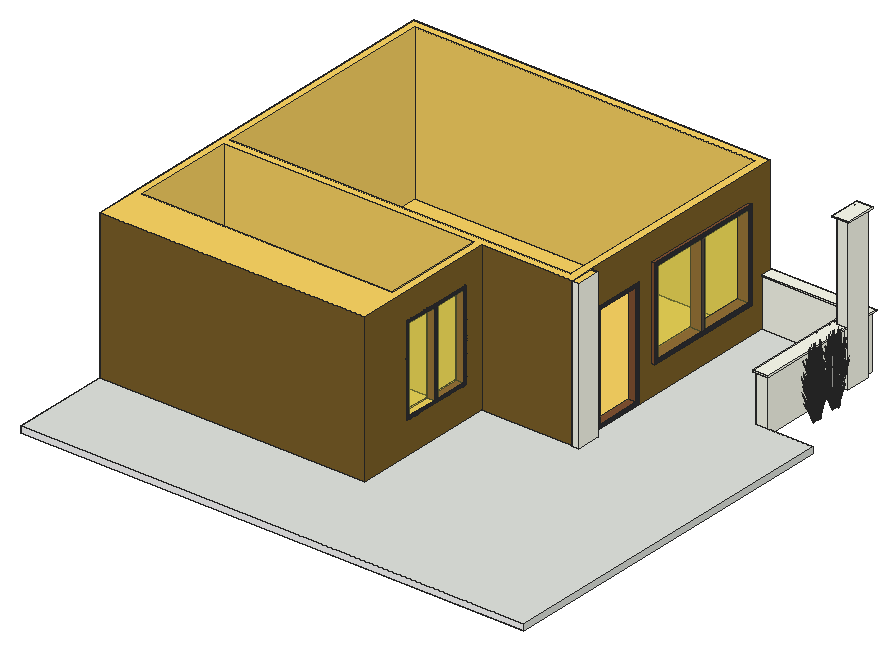
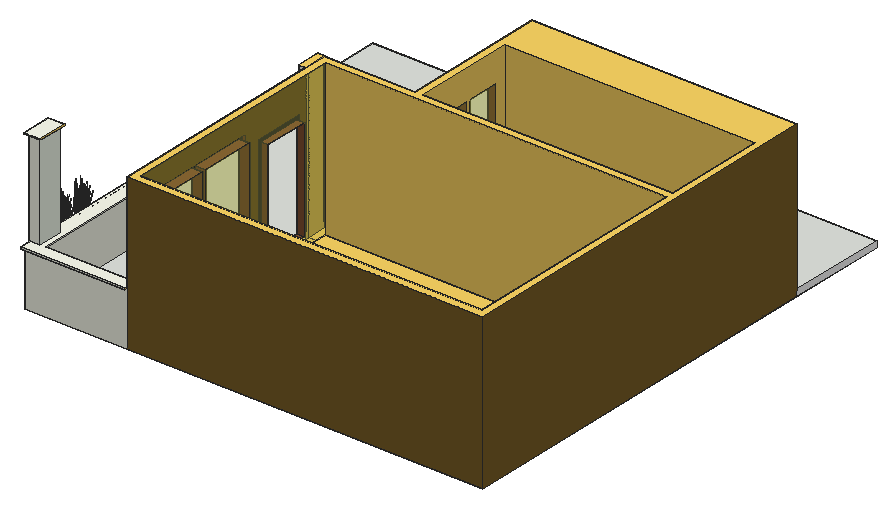
# SketchUp Ruby script. Lengths in inches.
U = 1.inch
M = Sketchup.active_model
def pt(a) = Geom::Point3d.new(a.map { |v| v * U })
def face(e, loops, mat)
  f = e.add_face(loops[0].map { |a| pt(a) })
  loops[1..].each { |l| e.add_face(l.map { |a| pt(a) }).erase! }
  f.material = f.back_material = mat if mat
  f
end
# faces: each face lists its corners as indices into pts; further lists are holes
def faces(e, pts, list, mat = nil) = list.each { |f| face(e, (f[0].is_a?(Array) ? f : [f]).map { |l| l.map { |i| pts[i] } }, mat) }
# xy, xz, yz: faces in a plane at the given z, y or x. An outline is a flat list of corners, or four numbers for a rectangle; further outlines are holes
def ring(l) = l.size == 4 ? [[l[0], l[1]], [l[2], l[1]], [l[2], l[3]], [l[0], l[3]]] : l.each_slice(2).to_a
def flat(e, list, mat, &to3) = list.each { |f| face(e, (f[0].is_a?(Array) ? f : [f]).map { |l| ring(l).map { |u, v| to3.(u, v) } }, mat) }
def xy(e, z, list, mat = nil) = flat(e, list, mat) { |x, y| [x, y, z] }
def xz(e, y, list, mat = nil) = flat(e, list, mat) { |x, z| [x, y, z] }
def yz(e, x, list, mat = nil) = flat(e, list, mat) { |y, z| [x, y, z] }
def lines(e, pts, list) = list.each { |a, b| e.add_line(pt(pts[a]), pt(pts[b])) }
# prism: a flat outline (further loops are holes) pulled along v
def prism(e, loops, v, mat = nil)
  f = face(e, loops, mat); d = Geom::Vector3d.new(v.map { |x| x * U })
  f.pushpull(f.normal.samedirection?(d) ? d.length : -d.length)
end
def box(e, o, s, mat = nil) = prism(e, [[o, [o[0] + s[0], o[1], o[2]], [o[0] + s[0], o[1] + s[1], o[2]], [o[0], o[1] + s[1], o[2]]]], [0, 0, s[2]], mat)
def at(x, y, z, deg = 0) = Geom::Transformation.translation(pt([x, y, z])) * Geom::Transformation.rotation(ORIGIN, Z_AXIS, deg.degrees)
def axes(o, x, y, z) = Geom::Transformation.new([*x, 0, *y, 0, *z, 0, *pt(o).to_a, 1])
def part(name) = M.definitions.add(name)
# library, detail: a bought-in or finely detailed component or shape, given as its bounding box
def library(name, o, s) = part(name).tap { |d| box(d.entities, o, s) }
def detail(e, o, s) = box(e.add_group.entities, o, s)
def put(e, d, t, mat = nil) = e.add_instance(d, t).tap { |i| i.material = mat if mat }
def group(e, t, mat = nil) = e.add_group.tap { |g| g.transformation = t; g.material = mat if mat }.entities
root = M.entities
M.materials.add("Asphalt_02_1K").color = [86, 76, 68]
M.materials.add("Concrete_04_1K").color = [254, 255, 241]
M.materials.add("D03_Lemon_Mist").color = [255, 216, 101]
M.materials.add("Glass_Basic_01").color = [253, 255, 84]
M.materials["Glass_Basic_01"].alpha = 0.25
M.materials.add("LightPink_Translucent").color = [144, 107, 117]
M.materials["LightPink_Translucent"].alpha = 0.75
M.materials.add("Marble_01_1K").color = [227, 230, 224]
M.materials.add("Plywood_01_1K").color = [130, 82, 50]
M.materials.add("Plywood_01_1K1").color = [125, 97, 41]
M.materials.add("Roofing_01_1K").color = [248, 255, 241]
M.materials.add("ThomThom - Buttons1").color = [48, 49, 53]
M.materials.add("[Color_000]").color = [255, 255, 255]
c1 = part("blade")
p = [[2.15,0.21,22],[0,0.17,0],[0.09,0.45,0],[2.18,0.31,22],[2.29,0.31,22],[0.38,0.45,0],
  [2.48,0.24,33],[2.49,0.24,33],[2.48,0.22,33]]
faces(c1.entities,p,[[0,1,2,3],[4,5,2,3],[6,3,4,7],[8,0,3,6]])
c2 = part("seeds")
p = [[0.3,-0.1,1.38],[-0.01,-0.03,1.59],[-0.01,-0.03,0.03],[0.14,-0.07,-0.07],[0.29,-0.03,3],[0.15,0.01,3.11]]
faces(c2.entities,p,[[0,1,2,3],[1,0,4,5]],"LightPink_Translucent")
c3 = part("blade with seeds")
put(c3.entities,c1,at(0,0,0))
put(c3.entities,c2,axes([2.4,0.25,30.99],[1.5799,-0.05474,1.17369],[-0.12525,1.92788,0.29478],[-0.07173,-0.02425,1.56792]))
g1 = group(root,at(15,107.18,0),"D03_Lemon_Mist")
xy(g1,-2,[[[9,-98.18,408,-98.18,408,187.71,372,187.71,372,263.71,375,263.71,375,283.71,372,283.71,372,291,9,291],[15,15,15,96,213,96,213,102,15,102,15,285,285,285,285,102,213,102,213,15]],[15,15,213,96],[15,102,285,285]])
xy(g1,3,[[9,-98.18,408,-98.18,408,187.71,363,187.71,363,283.71,291,283.71,291,114,297,114,297,95,291,95,291,96,219,96,219,-19.85,9,-19.85]],"Marble_01_1K")
xy(g1,6,[[285,123,291,159]],"Plywood_01_1K")
xy(g1,27,[[291,174,294,270]],"Plywood_01_1K")
xy(g1,30,[[213,24,219,49.5]])
xy(g1,30,[[213,52.5,219,78],[285,177,294,220.5],[285,223.5,294,267]],"Plywood_01_1K")
xy(g1,41,[[362,185.71,372,187.71],[372,185.71,374,263.71],[362,187.71,363,282.71],[291,282.71,363,283.71],[372,283.71,374,293],
  [291,291,372,293]])
xy(g1,42,[[362,185.71,374,185.71,374,263.71,366,263.71,366,283.71,374,283.71,374,293,291,293,291,282.71,362,282.71]],"Concrete_04_1K")
xy(g1,87,[[285,123,291,159]],"Plywood_01_1K")
xy(g1,96,[[213,24,219,49.5],[213,52.5,219,78],[285,177,294,220.5],[285,223.5,294,267]],"Plywood_01_1K")
xy(g1,99,[[291,174,294,270]],"Plywood_01_1K")
xy(g1,118,[[366,263.71,375,283.71]])
xy(g1,118,[[364,261.71,364,283.71,366,283.71,366,263.71,375,263.71,375,283.71,364,283.71,364,285.71,377,285.71,377,261.71]],"Concrete_04_1K")
xy(g1,119,[[364,261.71,377,285.71]],"Concrete_04_1K")
xy(g1,120,[[[9,-19.85,219,-19.85,219,96,291,96,291,291,9,291,9,15,15,15,15,96,213,96,213,15,9,15],[15,102,285,285]],[291,95,297,114]])
xz(g1,-98.18,[[9,-2,408,3]],"[Color_000]")
xz(g1,-19.85,[[9,3,219,120]],"Plywood_01_1K1")
xz(g1,15,[[15,-2,213,120]])
xz(g1,24,[[213,30,219,96]],"Plywood_01_1K")
xz(g1,49.5,[[213,30,219,96]],"Plywood_01_1K")
xz(g1,52.5,[[213,30,219,96]],"Plywood_01_1K")
xz(g1,78,[[213,30,219,96]],"Plywood_01_1K")
xz(g1,95,[[291,3,297,120]],"Concrete_04_1K")
xz(g1,96,[[15,-2,213,120]],"D03_Lemon_Mist")
xz(g1,96,[[219,3,291,120]],"Plywood_01_1K1")
xz(g1,102,[[15,-2,285,120]])
xz(g1,114,[[291,3,297,120]],"Concrete_04_1K")
xz(g1,123,[[285,6,291,87]],"Plywood_01_1K")
xz(g1,159,[[285,6,291,87]],"Plywood_01_1K")
xz(g1,174,[[291,27,294,99]],"Plywood_01_1K")
xz(g1,177,[[285,30,294,96]],"Plywood_01_1K")
xz(g1,185.71,[[362,41,374,42]],"Concrete_04_1K")
xz(g1,187.71,[[363,3,372,41]],"Concrete_04_1K")
xz(g1,187.71,[[372,-2,408,3]],"[Color_000]")
xz(g1,220.5,[[285,30,294,96]],"Plywood_01_1K")
xz(g1,223.5,[[285,30,294,96]],"Plywood_01_1K")
xz(g1,261.71,[[364,118,377,119]],"Concrete_04_1K")
xz(g1,263.71,[[372,-2,375,-2,375,118,366,118,366,42,374,42,374,41,372,41]],"Concrete_04_1K")
xz(g1,267,[[285,30,294,96]],"Plywood_01_1K")
xz(g1,270,[[291,27,294,99]],"Plywood_01_1K")
xz(g1,282.71,[[291,41,362,42]],"Concrete_04_1K")
xz(g1,283.71,[[372,-2,372,41,374,41,374,42,366,42,366,118,375,118,375,-2],[291,3,363,41]],"Concrete_04_1K")
xz(g1,285,[[15,-2,285,120]],"D03_Lemon_Mist")
xz(g1,285.71,[[364,118,377,119]])
xz(g1,291,[[291,-2,372,41]],"Concrete_04_1K")
xz(g1,291,[[9,-2,291,120]],"Plywood_01_1K1")
xz(g1,293,[[291,41,374,42]],"Concrete_04_1K")
yz(g1,9,[[-19.85,-2,291,120]],"Plywood_01_1K1")
yz(g1,9,[[-98.18,-2,-19.85,3]],"[Color_000]")
yz(g1,15,[[15,-2,96,120],[102,-2,285,120]],"D03_Lemon_Mist")
yz(g1,213,[[[15,-2,96,120],[24,30,49.5,96],[52.5,30,78,96]]])
yz(g1,213,[[24,30,49.5,96],[52.5,30,78,96]],"Glass_Basic_01")
yz(g1,219,[[24,30,49.5,96],[52.5,30,78,96]],"Glass_Basic_01")
yz(g1,219,[[[-19.85,3,96,120],[21,27,81,99]]],"Plywood_01_1K1")
yz(g1,219,[[[21,27,81,99],[52.5,30,78,96],[24,30,49.5,96]]],"ThomThom - Buttons1")
yz(g1,285,[[[102,-2,285,120],[123,6,159,87],[223.5,30,267,96],[177,30,220.5,96]],[177,30,220.5,96],[223.5,30,267,96]],"Glass_Basic_01")
yz(g1,291,[[96,-2,111,120],[111,-2,114,120],[291,41,293,42]])
yz(g1,291,[[95,3,96,120]],"Concrete_04_1K")
yz(g1,291,[[[114,3,120,3,120,90,162,90,162,3,283.71,3,283.71,41,282.71,41,282.71,42,291,42,291,120,114,120],[174,27,270,99]]],"Plywood_01_1K1")
yz(g1,291,[[120,3,162,3,162,90,159,90,159,6,123,6,123,87,159,87,159,90,120,90]],"ThomThom - Buttons1")
yz(g1,294,[[220.5,30,223.5,96]],"Asphalt_02_1K")
yz(g1,294,[[177,30,220.5,96],[223.5,30,267,96]],"Glass_Basic_01")
yz(g1,294,[[[174,27,270,99],[177,30,267,96]]],"ThomThom - Buttons1")
yz(g1,297,[[95,3,114,120]],"Concrete_04_1K")
yz(g1,362,[[185.71,41,282.71,42]],"Concrete_04_1K")
yz(g1,363,[[187.71,3,283.71,41]],"Concrete_04_1K")
yz(g1,364,[[261.71,118,285.71,119]])
yz(g1,366,[[263.71,42,283.71,118]],"Roofing_01_1K")
yz(g1,372,[[187.71,-2,263.71,41],[283.71,-2,291,41]],"Concrete_04_1K")
yz(g1,374,[[185.71,41,263.71,42],[283.71,41,293,42]],"Concrete_04_1K")
yz(g1,375,[[263.71,-2,283.71,118]],"Concrete_04_1K")
yz(g1,377,[[261.71,118,285.71,119]],"Concrete_04_1K")
yz(g1,408,[[-98.18,-2,187.71,3]],"Marble_01_1K")
p = [[15,15,0],[9,15,0],[363,283.71,-2],[363,283.71,3],[363,187.71,-2],[363,187.71,3],
  [297,114,-2],[297,114,3],[297,96,-2],[297,96,3],[219,96,0],[219,96,3],
  [285,111,-2],[291,111,-2]]
lines(g1,p,[[0,1],[2,3],[4,5],[6,7],[8,9],[10,11],[12,13]])
put(root,c3,axes([397.28,348.51,0.23],[0.13077,0.0453,1.22981],[0.08428,0.46268,-0.26449],[-0.17763,0.08661,0.52581]))
put(root,c3,axes([398.43,347.03,0.875],[0.10696,-0.07982,1.52275],[0.03688,0.55733,0.11917],[-0.23167,0.07395,0.54424]))
put(root,c3,axes([398.09,346.14,2.28],[-0.37615,-0.01329,-0.61099],[0.02526,-0.55946,0.07373],[-0.15935,-0.05904,0.8643]))
put(root,c3,axes([397.78,346.27,0.23],[0.07347,0.15363,1.22981],[-0.16929,0.41759,-0.26449],[-0.17383,-0.09981,0.52581]))
put(root,c3,axes([397.48,347.1,1.89],[-0.31272,-0.15393,-0.30456],[0.09121,-0.44909,0.39319],[-0.1259,0.04118,0.75234]))
put(root,c3,axes([397.7,347.33,2.03],[-0.10194,0.50193,-0.43945],[-0.34951,-0.17204,-0.34039],[-0.14072,0.04602,0.84085]))
put(root,c3,axes([397.96,346.25,2.03],[-0.27323,0.36552,-0.43945],[-0.23929,-0.38612,-0.34039],[-0.13882,-0.05561,0.84085]))
put(root,c3,axes([397.52,347.3,-0.72],[0.00954,0.08696,1.51654],[-0.19238,0.45414,-0.23168],[-0.13665,-0.02289,0.25832]))
put(root,c3,axes([397,349.48,0.38],[0.15682,-0.25009,0.9878],[0.06188,0.39591,0.72577],[-0.11333,0.07089,0.21757]))
put(root,c3,axes([397.86,345.91,1.89],[-0.2141,-0.34548,-0.30456],[0.24447,-0.32704,0.39319],[-0.12421,-0.04976,0.75234]))
put(root,c3,axes([397.6,348.4,1.89],[-0.32754,0.07886,-0.30456],[-0.08649,-0.45081,0.39319],[-0.09386,0.12109,0.75234]))
put(root,c3,axes([398.4375,328.36,0.23],[0.13077,0.0453,1.22981],[0.08428,0.46268,-0.26449],[-0.17763,0.08661,0.52581]))
put(root,c3,axes([397.42,349.74,-0.72],[0.05047,0.05513,1.51654],[0.08558,0.51079,-0.23168],[-0.11187,0.10892,0.25832]))
put(root,c3,axes([397.35,346.73,0.38],[0.24023,-0.03948,0.9878],[-0.15239,0.3479,0.72577],[-0.11872,-0.05219,0.21757]))
put(root,c3,axes([399.6,326.875,0.875],[0.10696,-0.07982,1.52275],[0.03688,0.55733,0.11917],[-0.23167,0.07395,0.54424]))
put(root,c3,axes([399.25,325.98,2.28],[-0.37615,-0.01329,-0.61099],[0.02526,-0.55946,0.07373],[-0.15935,-0.05904,0.8643]))
put(root,c3,axes([398.94,326.12,0.23],[0.07347,0.15363,1.22981],[-0.16929,0.41759,-0.26449],[-0.17383,-0.09981,0.52581]))
put(root,c3,axes([398.64,326.95,1.89],[-0.31272,-0.15393,-0.30456],[0.09121,-0.44909,0.39319],[-0.1259,0.04118,0.75234]))
put(root,c3,axes([397.87,348.45,2.03],[0.09666,0.50384,-0.43945],[-0.36608,0.08814,-0.34039],[-0.10491,0.13533,0.84085]))
put(root,c3,axes([398.86,327.18,2.03],[-0.10194,0.50193,-0.43945],[-0.34951,-0.17204,-0.34039],[-0.14072,0.04602,0.84085]))
put(root,c3,axes([398.78,348.09,-0.23],[-0.39143,-0.09047,-0.53624],[0.0826,-0.55804,-0.14074],[-0.11681,-0.06762,1.18365]))
put(root,c3,axes([399.12,326.1,2.03],[-0.27323,0.36552,-0.43945],[-0.23929,-0.38612,-0.34039],[-0.13882,-0.05561,0.84085]))
put(root,c3,axes([398.68,327.15,-0.72],[0.00954,0.08696,1.51654],[-0.19238,0.45414,-0.23168],[-0.13665,-0.02289,0.25832]))
put(root,c3,axes([398.74,345.48,2.28],[-0.32086,-0.26671,-0.61099],[0.22803,-0.46737,0.07373],[-0.11625,-0.15925,0.8643]))
put(root,c3,axes([398.59,345.49,2.03],[-0.37131,0.13117,-0.43945],[-0.06495,-0.49674,-0.34039],[-0.09973,-0.14235,0.84085]))
put(root,c3,axes([398.27,349.15,-0.26],[-0.35217,-0.2759,-0.427],[0.2105,-0.49473,0],[-0.08021,-0.06284,1.35453]))
put(root,c3,axes([398.17,329.33,0.38],[0.15682,-0.25009,0.9878],[0.06188,0.39591,0.72577],[-0.11333,0.07089,0.21757]))
put(root,c3,axes([398.11,345.04,-0.72],[-0.03645,0.07269,1.51654],[-0.36835,0.15672,-0.23168],[-0.08898,-0.14257,0.25832]))
put(root,c3,axes([398.48,349.48,0.04],[-0.23526,0.55293,0],[-0.3936,-0.30836,-0.44382],[-0.08964,-0.07023,1.40792]))
put(root,c3,axes([399.02,325.75,1.89],[-0.2141,-0.34548,-0.30456],[0.24447,-0.32704,0.39319],[-0.12421,-0.04976,0.75234]))
put(root,c3,axes([398.76,328.25,1.89],[-0.32754,0.07886,-0.30456],[-0.08649,-0.45081,0.39319],[-0.09386,0.12109,0.75234]))
put(root,c3,axes([398.58,329.58,-0.72],[0.05047,0.05513,1.51654],[0.08558,0.51079,-0.23168],[-0.11187,0.10892,0.25832]))
put(root,c3,axes([398.51,326.58,0.38],[0.24023,-0.03948,0.9878],[-0.15239,0.3479,0.72577],[-0.11872,-0.05219,0.21757]))
put(root,c3,axes([398.05,350.28,0.23],[0.11874,-0.08705,1.22981],[0.29317,0.26247,-0.26449],[-0.08726,0.22711,0.52581]))
put(root,c3,axes([397.88,345.32,-0.17],[-0.10855,0.45057,-0.03348],[-0.33409,-0.1386,-0.15179],[-0.05073,-0.0737,0.50065]))
put(root,c3,axes([398.38,344.75,0.23],[-0.02279,0.18051,1.22981],[-0.33311,0.15111,-0.26449],[-0.07787,-0.23331,0.52581]))
put(root,c3,axes([399.22,348.17,0.29],[-0.37992,0.36634,-0.25022],[-0.25264,-0.51764,-0.43002],[-0.09374,-0.05257,1.37348]))
put(root,c3,axes([398.63,345.125,1.89],[-0.05812,-0.44446,-0.30456],[0.33222,-0.11736,0.39319],[-0.08923,-0.12737,0.75234]))
put(root,c3,axes([397.7,347.375,0.04],[-0.47052,0,0],[0,-0.61671,-0.44382],[0,-0.14046,1.40792]))
put(root,c3,axes([398.36,348.94,-0.26],[-0.08839,-0.48081,-0.26641],[0.35106,-0.13653,0.26641],[-0.07077,-0.05545,1.19518]))
put(root,c3,axes([398.17,349.44,1.89],[-0.2546,0.29052,-0.30456],[-0.24101,-0.33173,0.39319],[-0.03667,0.16855,0.75234]))
put(root,c3,axes([399.03,328.3,2.03],[0.09666,0.50384,-0.43945],[-0.36608,0.08814,-0.34039],[-0.10491,0.13533,0.84085]))
put(root,c3,axes([399.48,348.57,-0.23],[-0.25345,0.41475,-0.53624],[-0.31485,-0.37608,-0.14074],[-0.10156,0.10346,1.18365]))
put(root,c3,axes([398.07,347.21,0],[-0.35001,0.46392,0.2645],[-0.35022,-0.45904,-0.31383],[-0.01222,-0.13174,1.41801]))
put(root,c3,axes([399.94,327.9375,-0.23],[-0.39143,-0.09047,-0.53624],[0.0826,-0.55804,-0.14074],[-0.11681,-0.06762,1.18365]))
put(root,c3,axes([399.51,348.49,0.86],[0.32517,0.22251,1.30084],[-0.31856,0.47936,0.51441],[-0.14269,-0.28411,1.09053]))
put(root,c3,axes([399.9,325.32,2.28],[-0.32086,-0.26671,-0.61099],[0.22803,-0.46737,0.07373],[-0.11625,-0.15925,0.8643]))
put(root,c3,axes([398.27,344.46,0.38],[0.19628,0.19205,0.9878],[-0.28586,0.11545,0.72577],[-0.06116,-0.1476,0.21757]))
put(root,c3,axes([399.65,348.34,0.12],[-0.36743,-0.44413,-0.21665],[0.30918,-0.49872,0.47412],[-0.09894,0.05195,1.44665]))
put(root,c3,axes([399.75,325.34,2.03],[-0.37131,0.13117,-0.43945],[-0.06495,-0.49674,-0.34039],[-0.09973,-0.14235,0.84085]))
put(root,c3,axes([398.98,347.91,-0.1],[-0.22605,-0.46315,-0.38476],[0.34239,-0.32614,0.18517],[-0.07315,-0.05731,1.23533]))
put(root,c3,axes([398.34,349.14,2.59],[-0.00979,0.51041,-0.6782],[-0.4123,-0.03428,0.08184],[-0.04351,0.21623,0.95938]))
put(root,c3,axes([398.33,350.57,0.38],[-0.00974,-0.3281,0.9878],[0.24334,0.23402,0.72577],[-0.04786,0.15639,0.21757]))
put(root,c3,axes([399.43,328.99,-0.26],[-0.35217,-0.2759,-0.427],[0.2105,-0.49473,0],[-0.08021,-0.06284,1.35453]))
put(root,c3,axes([399.27,324.88,-0.72],[-0.03645,0.07269,1.51654],[-0.36835,0.15672,-0.23168],[-0.08898,-0.14257,0.25832]))
put(root,c3,axes([399.46,348.25,-0.1],[-0.40861,0.03406,-0.38476],[-0.03695,-0.56543,0.18517],[-0.07315,0.05731,1.23533]))
put(root,c3,axes([399.64,329.33,0.04],[-0.23526,0.55293,0],[-0.3936,-0.30836,-0.44382],[-0.08964,-0.07023,1.40792]))
put(root,c3,axes([398.68,349.19,0.13],[0.35217,0.2759,0.427],[-0.2105,0.49473,0],[-0.08021,-0.06284,1.35453]))
put(root,c3,axes([398.2,349.85,0.89],[0.00827,-0.28486,1.32737],[0.37184,0.15046,0.18343],[-0.03222,0.30359,0.62678]))
put(root,c3,axes([399.01,348.18,0.1],[0.09973,-0.65385,-0.20149],[0.47288,0.11397,0.44093],[-0.08263,-0.0903,1.34539]))
put(root,c3,axes([399.1875,348.33,0.25],[-0.07259,0.49245,0.12452],[-0.35466,-0.08548,-0.35559],[-0.06454,-0.05057,1.09]))
put(root,c3,axes([399.21,330.13,0.23],[0.11874,-0.08705,1.22981],[0.29317,0.26247,-0.26449],[-0.08726,0.22711,0.52581]))
put(root,c3,axes([399.89,349.7,-0.26],[-0.35217,0.2759,-0.427],[-0.2105,-0.49473,0],[-0.08021,0.06284,1.35453]))
put(root,c3,axes([397.81,346.96,-0.26],[0,-0.5518,-0.427],[0.42099,0,0],[0,-0.12568,1.35453]))
put(root,c3,axes([399.04,325.16,-0.17],[-0.10855,0.45057,-0.03348],[-0.33409,-0.1386,-0.15179],[-0.05073,-0.0737,0.50065]))
put(root,c3,axes([397.99,347.47,0.13],[0,0.5518,0.427],[-0.42099,0,0],[0,-0.12568,1.35453]))
put(root,c3,axes([399.92,349.56,-0.11],[-0.23233,-0.55486,-0.04422],[0.3936,-0.30836,0.44382],[-0.09699,0.05283,1.40722]))
put(root,c3,axes([398.43,349.31,2.3],[0.26937,0.37076,-0.48779],[-0.28456,0.3247,-0.37783],[-0.04099,0.18838,0.93334]))
put(root,c3,axes([399.54,324.6,0.23],[-0.02279,0.18051,1.22981],[-0.33311,0.15111,-0.26449],[-0.07787,-0.23331,0.52581]))
put(root,c3,axes([399.81,349.49,-0.26],[-0.35106,-0.13653,-0.26641],[0.08839,-0.48081,0.26641],[-0.07077,0.05545,1.19518]))
put(root,c3,axes([400.38,328.02,0.29],[-0.37992,0.36634,-0.25022],[-0.25264,-0.51764,-0.43002],[-0.09374,-0.05257,1.37348]))
put(root,c3,axes([398.91,347.59,0.29],[-0.42377,-0.26329,-0.25022],[0.20405,-0.55571,-0.43002],[-0.01332,-0.13644,1.37348]))
put(root,c3,axes([400.01,347.43,0.44],[-0.01028,-0.51954,1.21494],[0.46521,0.13467,0.51441],[-0.11003,0.28429,1.14681]))
put(root,c3,axes([399.79,324.97,1.89],[-0.05812,-0.44446,-0.30456],[0.33222,-0.11736,0.39319],[-0.08923,-0.12737,0.75234]))
put(root,c3,axes([398.86,327.22,0.04],[-0.47052,0,0],[0,-0.61671,-0.44382],[0,-0.14046,1.40792]))
put(root,c3,axes([399.52,328.79,-0.26],[-0.08839,-0.48081,-0.26641],[0.35106,-0.13653,0.26641],[-0.07077,-0.05545,1.19518]))
put(root,c3,axes([398.13,349.86,0.43],[0.34184,-0.09771,0.05596],[0.07859,0.39367,-0.74222],[-0.02167,0.19928,0.6653]))
put(root,c3,axes([399.33,329.29,1.89],[-0.2546,0.29052,-0.30456],[-0.24101,-0.33173,0.39319],[-0.03667,0.16855,0.75234]))
put(root,c3,axes([399.75,348.09,0.29],[0.04385,0.62963,-0.25022],[-0.45669,0.03807,-0.43002],[-0.08042,0.08387,1.37348]))
put(root,c3,axes([398.72,347.03,-0.2],[-0.15453,-0.56584,-0.60058],[0.44514,-0.20379,-0.15763],[-0.01708,-0.19161,1.32568]))
put(root,c3,axes([399.41,345.26,2.03],[-0.3699,-0.13833,-0.43945],[0.12679,-0.47426,-0.34039],[-0.03392,-0.19095,0.84085]))
put(root,c3,axes([400.64,328.42,-0.23],[-0.25345,0.41475,-0.53624],[-0.31485,-0.37608,-0.14074],[-0.10156,0.10346,1.18365]))
put(root,c3,axes([397.99,346.97,-0.26],[0.26266,-0.34428,-0.26641],[0.26266,0.34428,0.26641],[0,-0.11089,1.19518]))
put(root,c3,axes([399.23,327.06,0],[-0.35001,0.46392,0.2645],[-0.35022,-0.45904,-0.31383],[-0.01222,-0.13174,1.41801]))
put(root,c3,axes([399.17,344.74,-0.17],[-0.26003,0.31656,-0.03348],[-0.23826,-0.3467,-0.15179],[-0.01677,-0.09824,0.50065]))
put(root,c3,axes([399.07,347.86,0.03],[0.4756,0.11626,0.39349],[-0.09679,0.6566,0.15441],[-0.0695,-0.0634,1.36617]))
put(root,c3,axes([400.67,328.34,0.86],[0.32517,0.22251,1.30084],[-0.31856,0.47936,0.51441],[-0.14269,-0.28411,1.09053]))
put(root,c3,axes([399.43,324.31,0.38],[0.19628,0.19205,0.9878],[-0.28586,0.11545,0.72577],[-0.06116,-0.1476,0.21757]))
put(root,c3,axes([400.8125,328.1875,0.12],[-0.36743,-0.44413,-0.21665],[0.30918,-0.49872,0.47412],[-0.09894,0.05195,1.44665]))
put(root,c3,axes([400.14,327.76,-0.1],[-0.22605,-0.46315,-0.38476],[0.34239,-0.32614,0.18517],[-0.07315,-0.05731,1.23533]))
put(root,c3,axes([398.95,347.74,0.34],[-0.18257,0.49721,0.38476],[-0.37935,-0.23929,-0.18517],[0,-0.11462,1.23533]))
put(root,c3,axes([399.55,345.35,2.28],[-0.17959,-0.44867,-0.61099],[0.36969,-0.25004,0.07373],[-0.042,-0.21679,0.8643]))
put(root,c3,axes([399.5,328.98,2.59],[-0.00979,0.51041,-0.6782],[-0.4123,-0.03428,0.08184],[-0.04351,0.21623,0.95938]))
put(root,c3,axes([399.5,330.42,0.38],[-0.00974,-0.3281,0.9878],[0.24334,0.23402,0.72577],[-0.04786,0.15639,0.21757]))
put(root,c3,axes([400.625,328.09,-0.1],[-0.40861,0.03406,-0.38476],[-0.03695,-0.56543,0.18517],[-0.07315,0.05731,1.23533]))
put(root,c3,axes([398.8125,348.91,0.13],[0.40434,-0.14646,0.15172],[0.09984,0.54504,0.30174],[-0.03606,-0.07941,1.3795]))
put(root,c3,axes([399.33,349,-0.11],[-0.37935,-0.24773,0],[0.18257,-0.51475,0],[0,0,1.39928]))
put(root,c3,axes([400.21,349.62,0.04],[0.23526,0.55293,0],[-0.3936,0.30836,-0.44382],[-0.08964,0.07023,1.40792]))
put(root,c3,axes([399.84,329.04,0.13],[0.35217,0.2759,0.427],[-0.2105,0.49473,0],[-0.08021,-0.06284,1.35453]))
put(root,c3,axes([399.37,329.7,0.89],[0.00827,-0.28486,1.32737],[0.37184,0.15046,0.18343],[-0.03222,0.30359,0.62678]))
put(root,c3,axes([400.18,328.03,0.1],[0.09973,-0.65385,-0.20149],[0.47288,0.11397,0.44093],[-0.08263,-0.0903,1.34539]))
put(root,c3,axes([400.35,328.18,0.25],[-0.07259,0.49245,0.12452],[-0.35466,-0.08548,-0.35559],[-0.06454,-0.05057,1.09]))
put(root,c3,axes([400.02,348.94,0.13],[0.1087,-0.54839,0.15172],[0.39778,0.15519,0.30174],[-0.06871,0.00267,1.3795]))
put(root,c3,axes([399.83,348.21,0.25],[0.278,0.33153,0.12452],[-0.23189,0.37404,-0.35559],[-0.06454,0.05057,1.09]))
put(root,c3,axes([401.05,329.55,-0.26],[-0.35217,0.2759,-0.427],[-0.2105,-0.49473,0],[-0.08021,0.06284,1.35453]))
put(root,c3,axes([398.97,326.8,-0.26],[0,-0.5518,-0.427],[0.42099,0,0],[0,-0.12568,1.35453]))
put(root,c3,axes([399.15,327.31,0.13],[0,0.5518,0.427],[-0.42099,0,0],[0,-0.12568,1.35453]))
put(root,c3,axes([401.08,329.4,-0.11],[-0.23233,-0.55486,-0.04422],[0.3936,-0.30836,0.44382],[-0.09699,0.05283,1.40722]))
put(root,c3,axes([399.73,347.81,-0.02],[-0.35001,-0.47494,-0.05273],[0.35022,-0.47523,0],[-0.01222,-0.01659,1.50991]))
put(root,c3,axes([399.83,347.97,0.34],[0.40861,-0.03406,0.38476],[0.03695,0.56543,-0.18517],[-0.07315,0.05731,1.23533]))
put(root,c3,axes([399.93,349.27,0],[0.47108,0.17935,0.2645],[-0.11785,0.64108,-0.31383],[-0.07797,0.08023,1.41801]))
put(root,c3,axes([399.59,329.15,2.3],[0.26937,0.37076,-0.48779],[-0.28456,0.3247,-0.37783],[-0.04099,0.18838,0.93334]))
put(root,c3,axes([399.24,344.35,-0.72],[-0.06312,0.01988,1.51654],[-0.34903,-0.22379,-0.23168],[0.00586,-0.18666,0.25832]))
put(root,c3,axes([400.97,329.33,-0.26],[-0.35106,-0.13653,-0.26641],[0.08839,-0.48081,0.26641],[-0.07077,0.05545,1.19518]))
put(root,c3,axes([400.13,349.24,0.13],[0.35217,-0.2759,0.427],[0.2105,0.49473,0],[-0.08021,0.06284,1.35453]))
put(root,c3,axes([400.07,327.44,0.29],[-0.42377,-0.26329,-0.25022],[0.20405,-0.55571,-0.43002],[-0.01332,-0.13644,1.37348]))
put(root,c3,axes([401.17,327.28,0.44],[-0.01028,-0.51954,1.21494],[0.46521,0.13467,0.51441],[-0.11003,0.28429,1.14681]))
put(root,c3,axes([399.58,344.97,1.89],[0.11344,-0.42434,-0.30456],[0.33096,0.12377,0.39319],[-0.03035,-0.17085,0.75234]))
put(root,c3,axes([399.03,347.26,0.03],[0.1636,0.61702,0.39349],[-0.46745,0.21456,0.15441],[0.00571,-0.11338,1.36617]))
put(root,c3,axes([398.95,347.18,-0.1],[0.18257,-0.49721,-0.38476],[0.37935,0.23929,0.18517],[0,-0.11462,1.23533]))
put(root,c3,axes([399.42,348.78,-0.1],[-0.12277,-0.47573,0],[0.35059,-0.1666,0],[0,0,1.32759]))
put(root,c3,axes([398.98,349.79,-0.72],[0.0609,-0.03003,1.51654],[0.36632,0.16527,-0.23168],[0.01071,0.18627,0.25832]))
put(root,c3,axes([399.06,349.96,1.89],[-0.11344,0.42434,-0.30456],[-0.33096,-0.12377,0.39319],[0.03035,0.17085,0.75234]))
put(root,c3,axes([399.29,329.71,0.43],[0.34184,-0.09771,0.05596],[0.07859,0.39367,-0.74222],[-0.02167,0.19928,0.6653]))
put(root,c3,axes([400.91,327.9375,0.29],[0.04385,0.62963,-0.25022],[-0.45669,0.03807,-0.43002],[-0.08042,0.08387,1.37348]))
put(root,c3,axes([399.88,326.88,-0.2],[-0.15453,-0.56584,-0.60058],[0.44514,-0.20379,-0.15763],[-0.01708,-0.19161,1.32568]))
put(root,c3,axes([400.58,325.11,2.03],[-0.3699,-0.13833,-0.43945],[0.12679,-0.47426,-0.34039],[-0.03392,-0.19095,0.84085]))
put(root,c3,axes([399.92,347.85,-0.1],[-0.18257,0.49721,-0.38476],[-0.37935,-0.23929,0.18517],[0,0.11462,1.23533]))
put(root,c3,axes([399.15,326.81,-0.26],[0.26266,-0.34428,-0.26641],[0.26266,0.34428,0.26641],[0,-0.11089,1.19518]))
put(root,c3,axes([400.34,324.59,-0.17],[-0.26003,0.31656,-0.03348],[-0.23826,-0.3467,-0.15179],[-0.01677,-0.09824,0.50065]))
put(root,c3,axes([400.23,327.71,0.03],[0.4756,0.11626,0.39349],[-0.09679,0.6566,0.15441],[-0.0695,-0.0634,1.36617]))
put(root,c3,axes([400.64,347.54,0.13],[-0.29564,-0.40194,0.15172],[0.29793,-0.38985,0.30174],[-0.03265,0.08208,1.3795]))
put(root,c3,axes([399.62,347.3125,-0.1],[0,-0.63847,0],[0.47052,0,0],[0,0,1.54332]))
put(root,c3,axes([399.18,347.43,0.09],[0.42398,0.26744,0.20696],[-0.20405,0.55571,0.43002],[0,-0.1281,1.38067]))
put(root,c3,axes([399.85,347.57,-0.03],[0,0.63816,-0.04848],[-0.47052,0,0],[0,0.02005,1.54256]))
put(root,c3,axes([400.11,327.59,0.34],[-0.18257,0.49721,0.38476],[-0.37935,-0.23929,-0.18517],[0,-0.11462,1.23533]))
put(root,c3,axes([400.71,325.2,2.28],[-0.17959,-0.44867,-0.61099],[0.36969,-0.25004,0.07373],[-0.042,-0.21679,0.8643]))
put(root,c3,axes([399.04,347.05,0.34],[-0.40861,0.03406,0.38476],[-0.03695,-0.56543,-0.18517],[0.07315,-0.05731,1.23533]))
put(root,c3,axes([398.85,346.08,0.13],[-0.1087,0.54839,0.15172],[-0.39778,-0.15519,0.30174],[0.06871,-0.00267,1.3795]))
put(root,c3,axes([399.63,348.8,-0.03],[0.1636,0.63392,-0.05171],[-0.46745,0.22213,0],[0.00571,0.02214,1.48069]))
put(root,c3,axes([399.98,328.76,0.13],[0.40434,-0.14646,0.15172],[0.09984,0.54504,0.30174],[-0.03606,-0.07941,1.3795]))
put(root,c3,axes([400.5,328.85,-0.11],[-0.37935,-0.24773,0],[0.18257,-0.51475,0],[0,0,1.39928]))
put(root,c3,axes([401.375,329.47,0.04],[0.23526,0.55293,0],[-0.3936,0.30836,-0.44382],[-0.08964,0.07023,1.40792]))
put(root,c3,axes([398.66,345.41,0.04],[-0.23526,-0.55293,0],[0.3936,-0.30836,-0.44382],[0.08964,-0.07023,1.40792]))
put(root,c3,axes([399.09,349.57,2.28],[0.17959,0.44867,-0.61099],[-0.36969,0.25004,0.07373],[0.042,0.21679,0.8643]))
put(root,c3,axes([400.98,347.97,-0.11],[-0.47029,-0.00441,-0.0428],[0,-0.61671,0.42951],[-0.01478,0.14039,1.36183]))
put(root,c3,axes([400.06,346.11,0.13],[-0.40434,0.14646,0.15172],[-0.09984,-0.54504,0.30174],[0.03606,0.07941,1.3795]))
put(root,c3,axes([401.18,328.79,0.13],[0.1087,-0.54839,0.15172],[0.39778,0.15519,0.30174],[-0.06871,0.00267,1.3795]))
put(root,c3,axes([399.64,344.07,0.38],[0.04827,0.32177,0.9878],[-0.26778,-0.17821,0.72577],[0.02882,-0.16476,0.21757]))
put(root,c3,axes([401,328.0625,0.25],[0.278,0.33153,0.12452],[-0.23189,0.37404,-0.35559],[-0.06454,0.05057,1.09]))
put(root,c3,axes([399.39,346.91,0.03],[-0.312,0.50076,0.39349],[-0.37066,-0.44204,0.15441],[0.07522,-0.04998,1.36617]))
put(root,c3,axes([400.9,327.65,-0.02],[-0.35001,-0.47494,-0.05273],[0.35022,-0.47523,0],[-0.01222,-0.01659,1.50991]))
put(root,c3,axes([399.93,347.7,-0.1],[0.26266,0.35642,0],[-0.26266,0.35642,0],[0,0,1.45569]))
put(root,c3,axes([400.99,327.82,0.34],[0.40861,-0.03406,0.38476],[0.03695,0.56543,-0.18517],[-0.07315,0.05731,1.23533]))
put(root,c3,axes([399.92,347.28,0.34],[0.18257,-0.49721,0.38476],[0.37935,0.23929,-0.18517],[0,0.11462,1.23533]))
put(root,c3,axes([399.77,349.01,-0.1],[0.37935,0.24773,0],[-0.18257,0.51475,0],[0,0,1.5046]))
put(root,c3,axes([401.09,329.12,0],[0.47108,0.17935,0.2645],[-0.11785,0.64108,-0.31383],[-0.07797,0.08023,1.41801]))
put(root,c3,axes([400.4,324.2,-0.72],[-0.06312,0.01988,1.51654],[-0.34903,-0.22379,-0.23168],[0.00586,-0.18666,0.25832]))
put(root,c3,axes([399.22,349.66,2.03],[0.3699,0.13833,-0.43945],[-0.12679,0.47426,-0.34039],[0.03392,0.19095,0.84085]))
put(root,c3,axes([401.29,329.08,0.13],[0.35217,-0.2759,0.427],[0.2105,0.49473,0],[-0.08021,0.06284,1.35453]))
put(root,c3,axes([399.8,347.16,0.05],[-0.4756,-0.11626,0.42311],[0.09679,-0.6566,0.16603],[0.0695,0.0634,1.46899]))
put(root,c3,axes([400.74,324.82,1.89],[0.11344,-0.42434,-0.30456],[0.33096,0.12377,0.39319],[-0.03035,-0.17085,0.75234]))
put(root,c3,axes([400.19,327.11,0.03],[0.1636,0.61702,0.39349],[-0.46745,0.21456,0.15441],[0.00571,-0.11338,1.36617]))
put(root,c3,axes([400.88,348.06,-0.26],[-0.26266,0.34428,-0.26641],[-0.26266,-0.34428,0.26641],[0,0.11089,1.19518]))
put(root,c3,axes([400.11,327.03,-0.1],[0.18257,-0.49721,-0.38476],[0.37935,0.23929,0.18517],[0,-0.11462,1.23533]))
put(root,c3,axes([400.58,328.63,-0.1],[-0.12277,-0.47573,0],[0.35059,-0.1666,0],[0,0,1.32759]))
put(root,c3,axes([400.14,329.63,-0.72],[0.0609,-0.03003,1.51654],[0.36632,0.16527,-0.23168],[0.01071,0.18627,0.25832]))
put(root,c3,axes([400.13,348,-0.2],[0.13798,0.50522,-0.59522],[-0.39745,0.18195,-0.15622],[0.01525,0.17108,1.31385]))
put(root,c3,axes([400.22,329.8,1.89],[-0.11344,0.42434,-0.30456],[-0.33096,-0.12377,0.39319],[0.03035,0.17085,0.75234]))
put(root,c3,axes([399.9375,347.45,-0.1],[0.42099,0,0],[0,0.57126,0],[0,0,1.5343]))
put(root,c3,axes([399.53,346.82,0.34],[-0.22605,-0.46315,0.38476],[0.34239,-0.32614,-0.18517],[0.07315,0.05731,1.23533]))
put(root,c3,axes([399.12,346.93,0.29],[-0.04385,-0.62963,-0.25022],[0.45669,-0.03807,-0.43002],[0.08042,-0.08387,1.37348]))
put(root,c3,axes([400.08,347.4,0.25],[0.35059,-0.16092,0.12452],[0.12277,0.45952,-0.35559],[0,0.10113,1.09]))
put(root,c3,axes([400.21,345.62,2.03],[-0.26937,-0.37076,-0.43945],[0.28456,-0.3247,-0.34039],[0.04099,-0.18838,0.84085]))
put(root,c3,axes([401.08,327.69,-0.1],[-0.18257,0.49721,-0.38476],[-0.37935,-0.23929,0.18517],[0,0.11462,1.23533]))
put(root,c3,axes([399.96,347.43,0.29],[0.42377,0.26329,-0.25022],[-0.20405,0.55571,-0.43002],[0.01332,0.13644,1.37348]))
put(root,c3,axes([399.06,345.54,-0.26],[0.35106,0.13653,-0.26641],[-0.08839,0.48081,0.26641],[0.07077,-0.05545,1.19518]))
put(root,c3,axes([401.8,327.39,0.13],[-0.29564,-0.40194,0.15172],[0.29793,-0.38985,0.30174],[-0.03265,0.08208,1.3795]))
put(root,c3,axes([400.78,327.16,-0.1],[0,-0.63847,0],[0.47052,0,0],[0,0,1.54332]))
put(root,c3,axes([400.04,344.96,0.23],[-0.10696,0.11169,1.22981],[-0.32033,-0.19549,-0.26449],[0.05938,-0.24312,0.52581]))
put(root,c3,axes([400.34,327.27,0.09],[0.42398,0.26744,0.20696],[-0.20405,0.55571,0.43002],[0,-0.1281,1.38067]))
put(root,c3,axes([401.01,327.41,-0.03],[0,0.63816,-0.04848],[-0.47052,0,0],[0,0.02005,1.54256]))
put(root,c3,axes([400.2,326.9,0.34],[-0.40861,0.03406,0.38476],[-0.03695,-0.56543,-0.18517],[0.07315,-0.05731,1.23533]))
put(root,c3,axes([400.88,347.56,0.13],[0,-0.5518,0.427],[0.42099,0,0],[0,0.12568,1.35453]))
put(root,c3,axes([401.0625,348.07,-0.26],[0,0.5518,-0.427],[-0.42099,0,0],[0,0.12568,1.35453]))
put(root,c3,axes([398.98,345.32,-0.26],[0.35217,-0.2759,-0.427],[0.2105,0.49473,0],[0.08021,-0.06284,1.35453]))
put(root,c3,axes([400.01,325.93,0.13],[-0.1087,0.54839,0.15172],[-0.39778,-0.15519,0.30174],[0.06871,-0.00267,1.3795]))
put(root,c3,axes([399.68,346.69,0.25],[0.07259,-0.49245,0.12452],[0.35466,0.08548,-0.35559],[0.06454,0.05057,1.09]))
put(root,c3,axes([400.79,328.65,-0.03],[0.1636,0.63392,-0.05171],[-0.46745,0.22213,0],[0.00571,0.02214,1.48069]))
put(root,c3,axes([400.1875,345.84,0.13],[-0.35217,-0.2759,0.427],[0.2105,-0.49473,0],[0.08021,0.06284,1.35453]))
put(root,c3,axes([400.3,345.79,2.28],[0.00979,-0.51041,-0.61099],[0.4123,0.03428,0.07373],[0.04351,-0.21623,0.8643]))
put(root,c3,axes([399.82,325.25,0.04],[-0.23526,-0.55293,0],[0.3936,-0.30836,-0.44382],[0.08964,-0.07023,1.40792]))
put(root,c3,axes([400.25,329.42,2.28],[0.17959,0.44867,-0.61099],[-0.36969,0.25004,0.07373],[0.042,0.21679,0.8643]))
